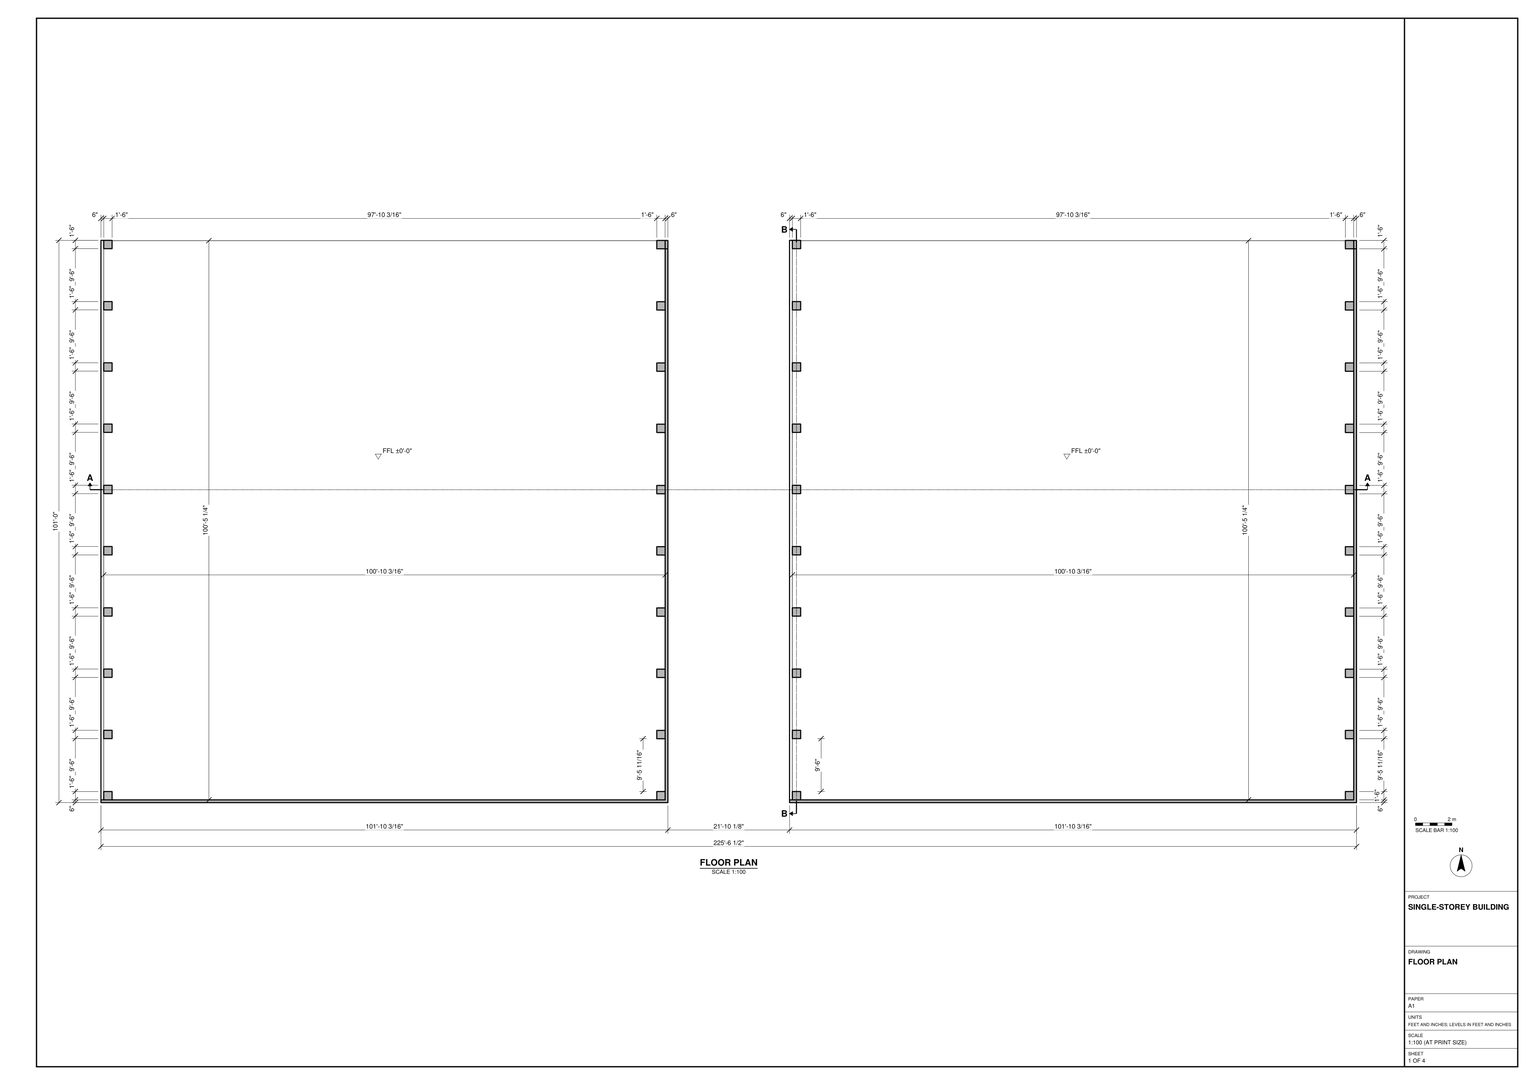
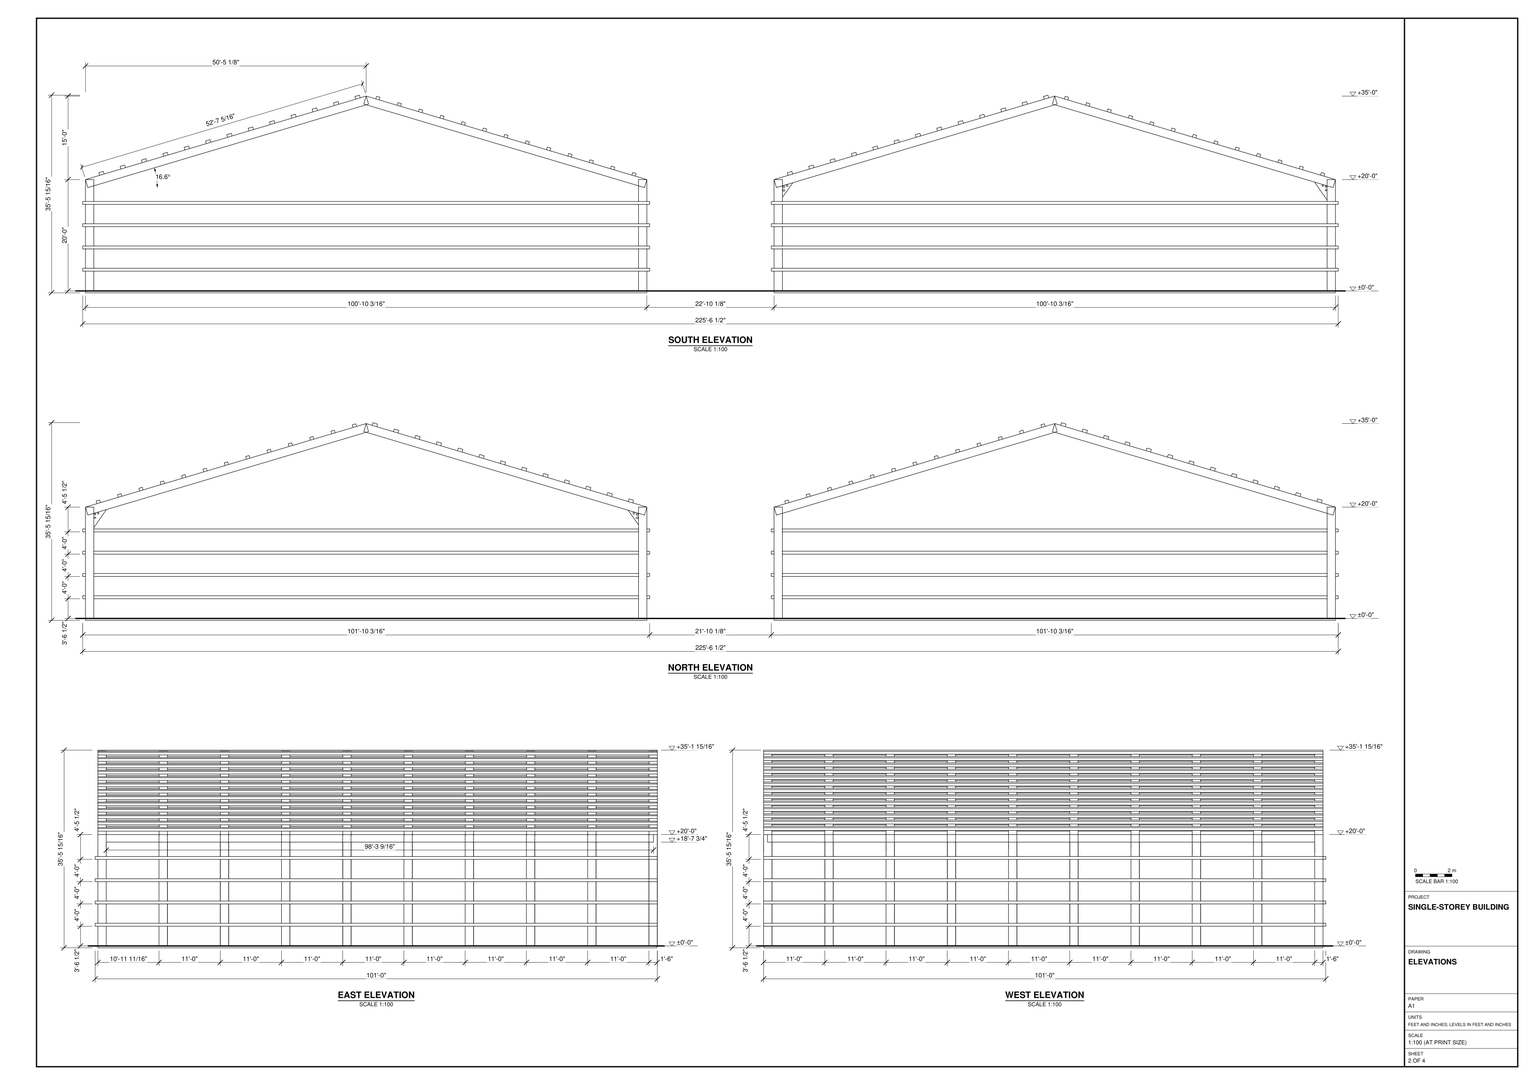
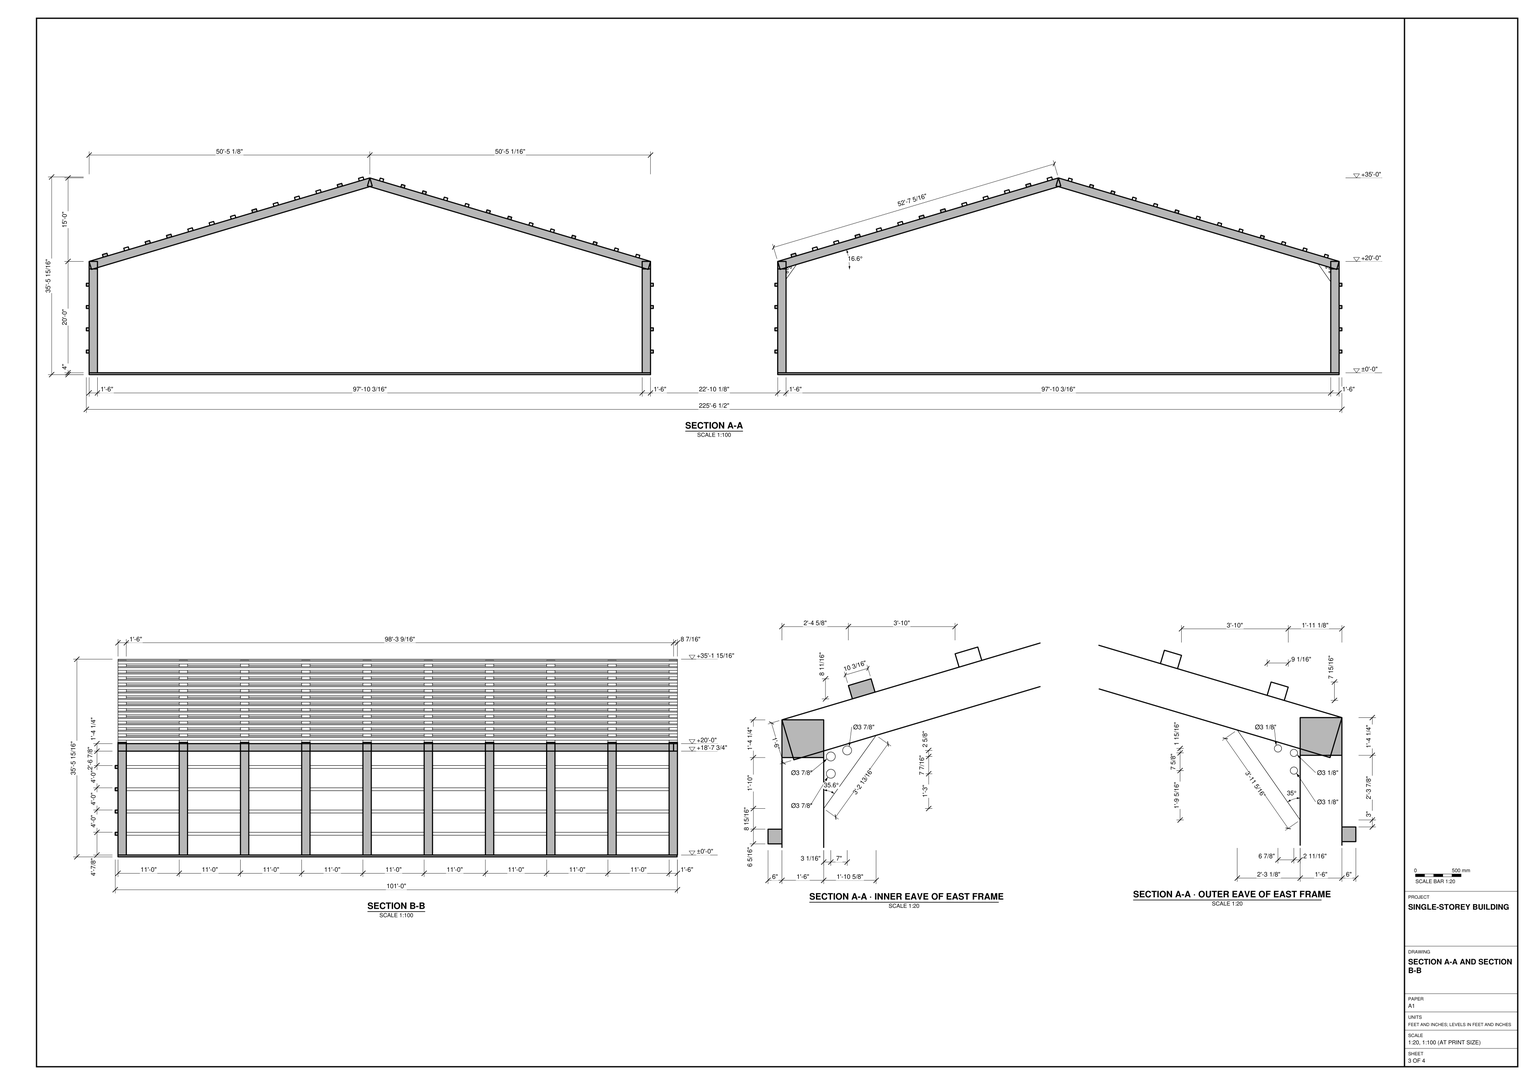
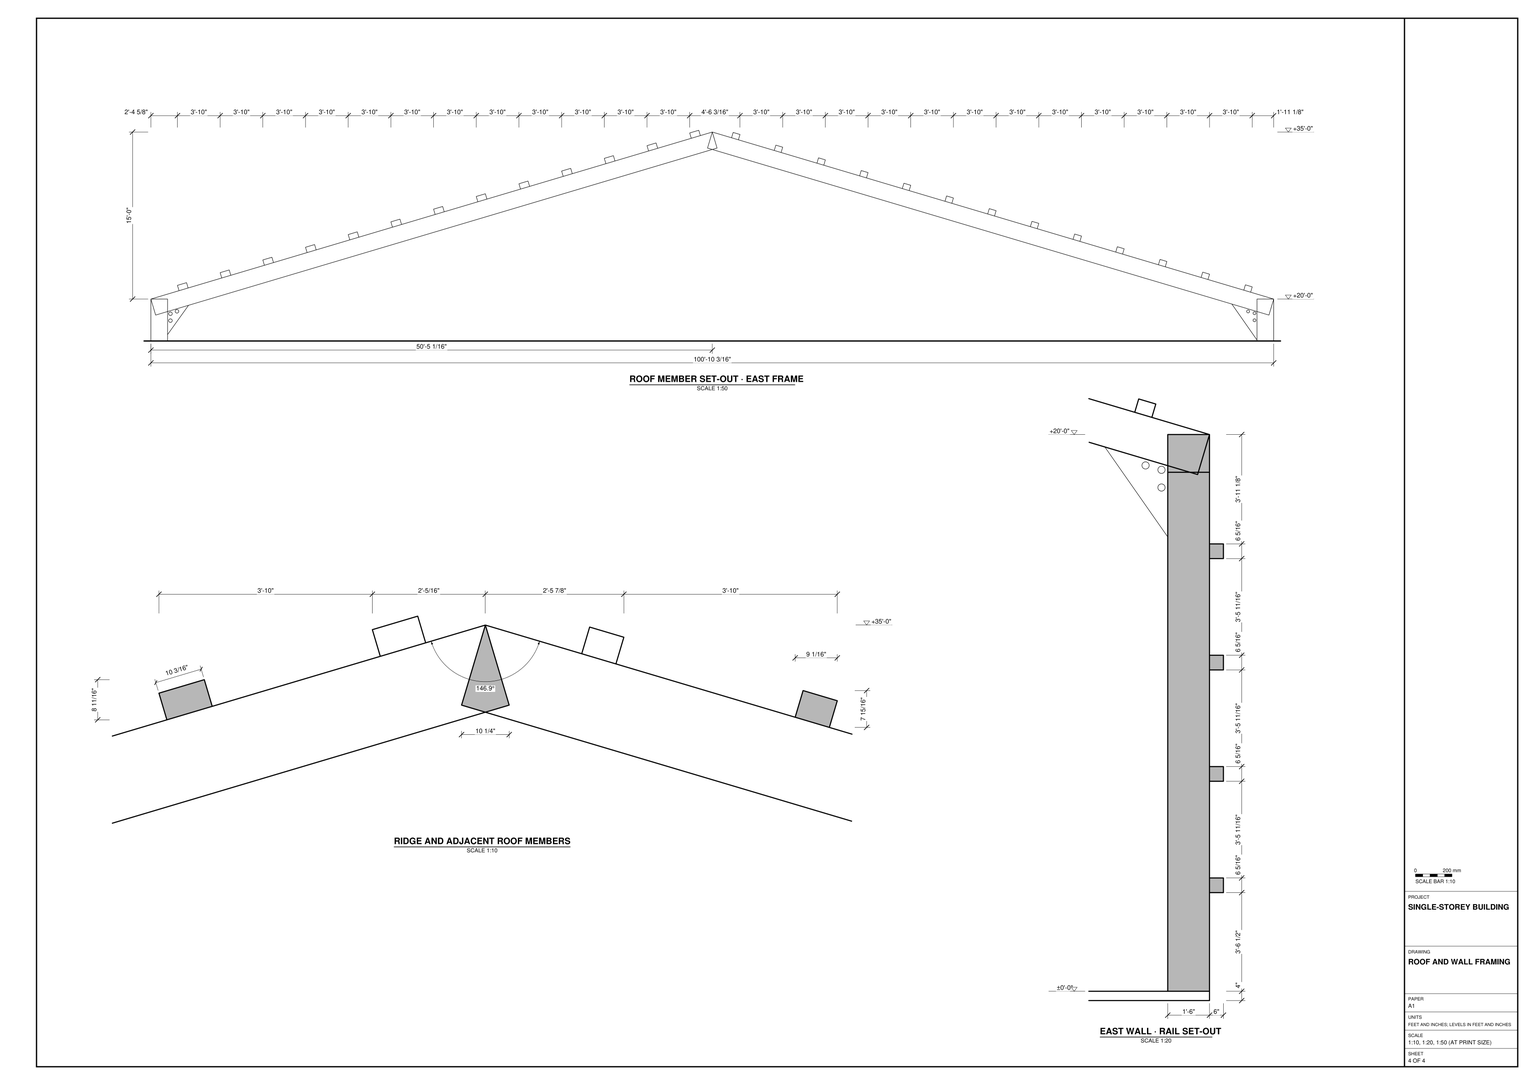
Build the two single-storey framed halls in SketchUp using task_files/diagram_01.pdf. Work in feet and inches. Set the finished floor of both halls at ±0'-0". The overall model must measure 225'-6 1/2" east to west, 101'-0" north to south and 35'-5 15/16" from its lowest to its highest point.

Lay out the two rectangular floor slabs side by side, with their north and south ends aligned. Leave the 21'-10 1/8" gap shown in plan between the halls. Keep each floor clear of interior partitions and columns. Along the east and west sides of each hall, place the paired columns at the bay spacing shown. Connect each pair with sloping rafters that meet at the ridge. Use the sections to size the framing and to distinguish the braced eave joints from the plain joints. Model the horizontal wall rails and the roof purlins as members with the cross-sections shown, leaving the spaces between them open.

Keep the slabs, wall framing and roof framing in separate groups or components, and use components for repeated members. Any decor or loose items shown may use suitable library components. Save one SketchUp model as output_files/two_single_storey_halls_with_exposed_gable_roof_framing.skp.

# SketchUp Ruby script. Lengths in inches.
U = 1.inch
M = Sketchup.active_model
def pt(a) = Geom::Point3d.new(a.map { |v| v * U })
def face(e, loops, mat)
  f = e.add_face(loops[0].map { |a| pt(a) })
  loops[1..].each { |l| e.add_face(l.map { |a| pt(a) }).erase! }
  f.material = f.back_material = mat if mat
  f
end
# faces: each face lists its corners as indices into pts; further lists are holes
def faces(e, pts, list, mat = nil) = list.each { |f| face(e, (f[0].is_a?(Array) ? f : [f]).map { |l| l.map { |i| pts[i] } }, mat) }
# xy, xz, yz: faces in a plane at the given z, y or x. An outline is a flat list of corners, or four numbers for a rectangle; further outlines are holes
def ring(l) = l.size == 4 ? [[l[0], l[1]], [l[2], l[1]], [l[2], l[3]], [l[0], l[3]]] : l.each_slice(2).to_a
def flat(e, list, mat, &to3) = list.each { |f| face(e, (f[0].is_a?(Array) ? f : [f]).map { |l| ring(l).map { |u, v| to3.(u, v) } }, mat) }
def xy(e, z, list, mat = nil) = flat(e, list, mat) { |x, y| [x, y, z] }
def xz(e, y, list, mat = nil) = flat(e, list, mat) { |x, z| [x, y, z] }
def yz(e, x, list, mat = nil) = flat(e, list, mat) { |y, z| [x, y, z] }
def lines(e, pts, list) = list.each { |a, b| e.add_line(pt(pts[a]), pt(pts[b])) }
# prism: a flat outline (further loops are holes) pulled along v
def prism(e, loops, v, mat = nil)
  f = face(e, loops, mat); d = Geom::Vector3d.new(v.map { |x| x * U })
  f.pushpull(f.normal.samedirection?(d) ? d.length : -d.length)
end
def box(e, o, s, mat = nil) = prism(e, [[o, [o[0] + s[0], o[1], o[2]], [o[0] + s[0], o[1] + s[1], o[2]], [o[0], o[1] + s[1], o[2]]]], [0, 0, s[2]], mat)
def at(x, y, z, deg = 0) = Geom::Transformation.translation(pt([x, y, z])) * Geom::Transformation.rotation(ORIGIN, Z_AXIS, deg.degrees)
def axes(o, x, y, z) = Geom::Transformation.new([*x, 0, *y, 0, *z, 0, *pt(o).to_a, 1])
def part(name) = M.definitions.add(name)
# library, detail: a bought-in or finely detailed component or shape, given as its bounding box
def library(name, o, s) = part(name).tap { |d| box(d.entities, o, s) }
def detail(e, o, s) = box(e.add_group.entities, o, s)
def put(e, d, t, mat = nil) = e.add_instance(d, t).tap { |i| i.material = mat if mat }
def group(e, t, mat = nil) = e.add_group.tap { |g| g.transformation = t; g.material = mat if mat }.entities
root = M.entities
M.materials.add("[Aluminum]").color = [179, 179, 179]
M.materials.add("[Terrazzo Tile Accent]").color = [224, 221, 217]
c1 = part("Group\#1")
box(c1.entities,[0,0,0],[1210.1875,1205.25,4])
c2 = part("Group\#2")
box(c2.entities,[0,0,0],[18,18,240])
c3 = part("Group\#3")
box(c3.entities,[0,0,0],[18,18,240])
c4 = part("Group\#4")
box(c4.entities,[0,0,0],[18,18,240])
c5 = part("Group\#5")
box(c5.entities,[0,0,0],[18,18,240])
c6 = part("Group\#6")
box(c6.entities,[0,0,0],[18,18,240])
c7 = part("Group\#7")
box(c7.entities,[0,0,0],[18,18,240])
c8 = part("Group\#8")
box(c8.entities,[0,0,0],[18,18,240])
c9 = part("Group\#9")
box(c9.entities,[0,0,0],[18,18,240])
c10 = part("Group\#10")
box(c10.entities,[0,0,0],[18,18,240])
c11 = part("Group\#11")
box(c11.entities,[0,0,0],[18,18,240])
c12 = part("Group\#12")
xz(c12.entities,0,[[5.13,0,605.09,178.47,599.96,180,605.09,197.25,0,17.25],[1205.06,0,1210.1875,17.25,605.09,197.25,610.23,180,605.09,178.47],[605.09,178.47,610.23,180,605.09,197.25,599.96,180]])
xz(c12.entities,18,[[5.13,0,0,17.25,605.09,197.25,599.96,180,605.09,178.47],[1205.06,0,605.09,178.47,610.23,180,605.09,197.25,1210.1875,17.25],[605.09,178.47,599.96,180,605.09,197.25,610.23,180]])
p = [[0,0,17.25],[0,18,17.25],[5.13,18,0],[5.13,0,0],[605.09,18,178.47],[610.23,18,180],
  [610.23,0,180],[605.09,0,178.47],[599.96,18,180],[1205.06,18,0],[1205.06,0,0],[599.96,0,180],
  [1210.1875,18,17.25],[1210.1875,0,17.25],[605.09,0,197.25],[605.09,18,197.25]]
faces(c12.entities,p,[[0,1,2,3],[3,2,4,5,6,7],[8,4,9,10,7,11],[12,13,10,9],[1,0,14,15],[12,15,14,13],[14,15,8,11],[15,14,6,5]])
c13 = part("Group\#13")
box(c13.entities,[0,0,0],[18,1179.59,16.27])
c14 = part("Group\#39")
prism(c14.entities,[[[1.71,1206,0],[1.71,0,0],[0,0,5.75],[0,1206,5.75]]],[9.78,0,2.91])
c15 = part("Group\#38")
prism(c15.entities,[[[1.71,1206,0],[1.71,0,0],[0,0,5.75],[0,1206,5.75]]],[9.78,0,2.91])
c16 = part("Group\#37")
prism(c16.entities,[[[1.71,1206,0],[1.71,0,0],[0,0,5.75],[0,1206,5.75]]],[9.78,0,2.91])
c17 = part("Group\#36")
prism(c17.entities,[[[1.71,1206,0],[1.71,0,0],[0,0,5.75],[0,1206,5.75]]],[9.78,0,2.91])
c18 = part("Group\#35")
prism(c18.entities,[[[1.71,1206,0],[1.71,0,0],[0,0,5.75],[0,1206,5.75]]],[9.78,0,2.91])
c19 = part("Group\#34")
prism(c19.entities,[[[1.71,1206,0],[1.71,0,0],[0,0,5.75],[0,1206,5.75]]],[9.78,0,2.91])
c20 = part("Group\#33")
prism(c20.entities,[[[1.71,1206,0],[1.71,0,0],[0,0,5.75],[0,1206,5.75]]],[9.78,0,2.91])
c21 = part("Group\#32")
prism(c21.entities,[[[1.71,1206,0],[1.71,0,0],[0,0,5.75],[0,1206,5.75]]],[9.78,0,2.91])
c22 = part("Group\#31")
prism(c22.entities,[[[1.71,1206,0],[1.71,0,0],[0,0,5.75],[0,1206,5.75]]],[9.78,0,2.91])
c23 = part("Group\#30")
prism(c23.entities,[[[1.71,1206,0],[1.71,0,0],[0,0,5.75],[0,1206,5.75]]],[9.78,0,2.91])
c24 = part("Group\#29")
prism(c24.entities,[[[1.71,1206,0],[1.71,0,0],[0,0,5.75],[0,1206,5.75]]],[9.78,0,2.91])
c25 = part("Group\#28")
prism(c25.entities,[[[1.71,1206,0],[1.71,0,0],[0,0,5.75],[0,1206,5.75]]],[9.78,0,2.91])
c26 = part("Group\#14")
prism(c26.entities,[[[1.71,1206,0],[1.71,0,0],[0,0,5.75],[0,1206,5.75]]],[9.78,0,2.91])
c27 = part("Group\#15")
prism(c27.entities,[[[0,1206,2.19],[7.37,1206,0],[7.37,0,0],[0,0,2.19]]],[1.71,0,5.75])
c28 = part("Group\#16")
prism(c28.entities,[[[0,1206,2.19],[7.37,1206,0],[7.37,0,0],[0,0,2.19]]],[1.71,0,5.75])
c29 = part("Group\#17")
prism(c29.entities,[[[0,1206,2.19],[7.37,1206,0],[7.37,0,0],[0,0,2.19]]],[1.71,0,5.75])
c30 = part("Group\#18")
prism(c30.entities,[[[0,1206,2.19],[7.37,1206,0],[7.37,0,0],[0,0,2.19]]],[1.71,0,5.75])
c31 = part("Group\#19")
prism(c31.entities,[[[0,1206,2.19],[7.37,1206,0],[7.37,0,0],[0,0,2.19]]],[1.71,0,5.75])
c32 = part("Group\#20")
prism(c32.entities,[[[0,1206,2.19],[7.37,1206,0],[7.37,0,0],[0,0,2.19]]],[1.71,0,5.75])
c33 = part("Group\#21")
prism(c33.entities,[[[0,1206,2.19],[7.37,1206,0],[7.37,0,0],[0,0,2.19]]],[1.71,0,5.75])
c34 = part("Group\#22")
prism(c34.entities,[[[0,1206,2.19],[7.37,1206,0],[7.37,0,0],[0,0,2.19]]],[1.71,0,5.75])
c35 = part("Group\#23")
prism(c35.entities,[[[0,1206,2.19],[7.37,1206,0],[7.37,0,0],[0,0,2.19]]],[1.71,0,5.75])
c36 = part("Group\#24")
prism(c36.entities,[[[0,1206,2.19],[7.37,1206,0],[7.37,0,0],[0,0,2.19]]],[1.71,0,5.75])
c37 = part("Group\#25")
prism(c37.entities,[[[0,1206,2.19],[7.37,1206,0],[7.37,0,0],[0,0,2.19]]],[1.71,0,5.75])
c38 = part("Group\#26")
prism(c38.entities,[[[0,1206,2.19],[7.37,1206,0],[7.37,0,0],[0,0,2.19]]],[1.71,0,5.75])
c39 = part("Group\#27")
prism(c39.entities,[[[0,1206,2.19],[7.37,1206,0],[7.37,0,0],[0,0,2.19]]],[1.71,0,5.75])
c40 = part("Group\#40")
yz(c40.entities,0,[[0,0,18,6.33]])
c41 = part("Group\#49")
g1 = group(c41.entities,at(0,0,0))
xy(g1,0,[[0,0,6,18]])
xy(g1,6.33,[[0,0,6,18]])
xz(g1,0,[[0,0,6,6.33]])
xz(g1,18,[[0,0,6,6.33]])
yz(g1,0,[[0,0,18,6.33]])
put(c41.entities,c40,at(6,0,0))
c42 = part("Group\#51")
g2 = group(c42.entities,at(0,0,0))
xy(g2,0,[[0,0,6,18]])
xy(g2,6.33,[[0,0,6,18]])
xz(g2,0,[[0,0,6,6.33]])
xz(g2,18,[[0,0,6,6.33]])
yz(g2,0,[[0,0,18,6.33]])
put(c42.entities,c40,at(6,0,0))
c43 = part("Group\#53")
g3 = group(c43.entities,at(0,0,0))
xy(g3,0,[[0,0,6,18]])
xy(g3,6.33,[[0,0,6,18]])
xz(g3,0,[[0,0,6,6.33]])
xz(g3,18,[[0,0,6,6.33]])
yz(g3,0,[[0,0,18,6.33]])
put(c43.entities,c40,at(6,0,0))
c44 = part("Group\#42")
g4 = group(c44.entities,at(0,0,0))
xy(g4,0,[[0,-1188,6,18]])
xy(g4,6.33,[[0,-1188,6,18]])
xz(g4,-1188,[[0,0,6,6.33]])
xz(g4,18,[[0,0,6,6.33]])
yz(g4,0,[[-1188,0,18,6.33]])
put(c44.entities,c40,at(6,0,0))
c45 = part("Group\#43")
g5 = group(c45.entities,at(0,0,0))
xy(g5,0,[[0,-1188,6,18]])
xy(g5,6.33,[[0,-1188,6,18]])
xz(g5,-1188,[[0,0,6,6.33]])
xz(g5,18,[[0,0,6,6.33]])
yz(g5,0,[[-1188,0,18,6.33]])
put(c45.entities,c40,at(6,0,0))
c46 = part("Group\#45")
g6 = group(c46.entities,at(0,0,0))
xy(g6,0,[[0,-1188,6,18]])
xy(g6,6.33,[[0,-1188,6,18]])
xz(g6,-1188,[[0,0,6,6.33]])
xz(g6,18,[[0,0,6,6.33]])
yz(g6,0,[[-1188,0,18,6.33]])
put(c46.entities,c40,at(6,0,0))
c47 = part("Group\#47")
g7 = group(c47.entities,at(0,0,0))
xy(g7,0,[[0,-1188,6,18]])
xy(g7,6.33,[[0,-1188,6,18]])
xz(g7,-1188,[[0,0,6,6.33]])
xz(g7,18,[[0,0,6,6.33]])
yz(g7,0,[[-1188,0,18,6.33]])
put(c47.entities,c40,at(6,0,0))
c48 = part("Group\#55")
p = [[27.12,0,30.73],[27.12,0,0],[0,0.28,38.8],[24.42,0.03,27.37],[24.82,0.02,27.43],[25.2,0.02,27.58],
  [25.52,0.02,27.83],[25.77,0.01,28.15],[25.93,0.01,28.53],[25.98,0.01,28.93],[25.93,0.01,29.34],[25.77,0.01,29.72],
  [25.52,0.02,30.04],[25.2,0.02,30.29],[24.82,0.02,30.44],[24.42,0.03,30.5],[24.01,0.03,30.44],[23.64,0.04,30.29],
  [23.3125,0.04,30.04],[23.06,0.04,29.72],[22.91,0.04,29.34],[22.86,0.04,28.93],[22.91,0.04,28.53],[23.06,0.04,28.15],
  [23.3125,0.04,27.83],[23.64,0.04,27.58],[24.01,0.03,27.43],[16.04,0.12,31.25],[15.99,0.12,30.84],[16.04,0.12,30.4375],
  [16.2,0.11,30.0625],[16.45,0.11,29.74],[16.77,0.11,29.49],[17.15,0.1,29.33],[17.55,0.1,29.28],[17.96,0.1,29.33],
  [18.33,0.09,29.49],[18.66,0.09,29.74],[18.91,0.09,30.0625],[19.0625,0.08,30.4375],[19.12,0.08,30.84],[19.0625,0.08,31.25],
  [18.91,0.09,31.625],[18.66,0.09,31.95],[18.33,0.09,32.2],[17.96,0.1,32.35],[17.55,0.1,32.4],[17.15,0.1,32.35],
  [16.77,0.11,32.2],[16.45,0.11,31.95],[16.2,0.11,31.625],[22.91,0.04,21.71],[22.86,0.04,21.31],[22.91,0.04,20.91],
  [23.06,0.04,20.53],[23.3125,0.04,20.2],[23.64,0.04,19.96],[24.01,0.03,19.8],[24.42,0.03,19.75],[24.82,0.02,19.8],
  [25.2,0.02,19.96],[25.52,0.02,20.2],[25.77,0.01,20.53],[25.93,0.01,20.91],[25.98,0.01,21.31],[25.93,0.01,21.71],
  [25.77,0.01,22.09],[25.52,0.02,22.41],[25.2,0.02,22.66],[24.82,0.02,22.82],[24.42,0.03,22.87],[24.01,0.03,22.82],
  [23.64,0.04,22.66],[23.3125,0.04,22.41],[23.06,0.04,22.09]]
faces(c48.entities,p,[[[0,1,2],[3,4,5,6,7,8,9,10,11,12,13,14,15,16,17,18,19,20,21,22,23,24,25,26],[27,28,29,30,31,32,33,34,35,36,37,38,39,40,41,42,43,44,45,46,47,48,49,50],[51,52,53,54,55,56,57,58,59,60,61,62,63,64,65,66,67,68,69,70,71,72,73,74]],[59,58,57,56,55,54,53,52,51,74,73,72,71,70,69,68,67,66,65,64,63,62,61,60],[4,3,26,25,24,23,22,21,20,19,18,17,16,15,14,13,12,11,10,9,8,7,6,5],[35,34,33,32,31,30,29,28,27,50,49,48,47,46,45,44,43,42,41,40,39,38,37,36]])
c49 = part("Group\#56")
xz(c49.entities,0,[[[0,0,0,24.82,22.6,31.54],[3.15,20.51,3.65,20.59,4.11,20.8,4.5,21.12,4.79,21.53,4.97,22,5.02,22.51,4.93,23.01,4.73,23.47,4.4,23.86,3.99,24.15,3.52,24.33,3.02,24.38,2.52,24.3,2.06,24.09,1.67,23.77,1.37,23.35,1.19,22.88,1.14,22.38,1.23,21.88,1.4375,21.42,1.76,21.03,2.17,20.73,2.64,20.56],[3.15,13.07,3.65,13.15,4.11,13.36,4.5,13.68,4.79,14.09,4.97,14.57,5.02,15.07,4.93,15.57,4.73,16.03,4.4,16.42,3.99,16.71,3.52,16.89,3.02,16.94,2.52,16.86,2.06,16.65,1.67,16.33,1.37,15.92,1.19,15.44,1.14,14.94,1.23,14.44,1.4375,13.98,1.76,13.59,2.17,13.3,2.64,13.12],[10.18,23.12,10.67,23.21,11.13,23.42,11.53,23.74,11.82,24.15,12,24.62,12.05,25.125,11.96,25.625,11.75,26.08,11.43,26.47,11.02,26.77,10.55,26.95,10.04,27,9.55,26.91,9.08,26.7,8.69,26.38,8.4,25.97,8.22,25.5,8.17,24.99,8.26,24.49,8.47,24.03,8.79,23.64,9.2,23.35,9.67,23.17]],[3.15,13.07,2.64,13.12,2.17,13.3,1.76,13.59,1.4375,13.98,1.23,14.44,1.14,14.94,1.19,15.44,1.37,15.92,1.67,16.33,2.06,16.65,2.52,16.86,3.02,16.94,3.52,16.89,3.99,16.71,4.4,16.42,4.73,16.03,4.93,15.57,5.02,15.07,4.97,14.57,4.79,14.09,4.5,13.68,4.11,13.36,3.65,13.15],[3.15,20.51,2.64,20.56,2.17,20.73,1.76,21.03,1.4375,21.42,1.23,21.88,1.14,22.38,1.19,22.88,1.37,23.35,1.67,23.77,2.06,24.09,2.52,24.3,3.02,24.38,3.52,24.33,3.99,24.15,4.4,23.86,4.73,23.47,4.93,23.01,5.02,22.51,4.97,22,4.79,21.53,4.5,21.12,4.11,20.8,3.65,20.59],[10.18,23.12,9.67,23.17,9.2,23.35,8.79,23.64,8.47,24.03,8.26,24.49,8.17,24.99,8.22,25.5,8.4,25.97,8.69,26.38,9.08,26.7,9.55,26.91,10.04,27,10.55,26.95,11.02,26.77,11.43,26.47,11.75,26.08,11.96,25.625,12.05,25.125,12,24.62,11.82,24.15,11.53,23.74,11.13,23.42,10.67,23.21]])
xy(root,46.52,[[0,0,0,6,1216.1875,6,1216.1875,1193.72,1222.1875,1193.72,1222.1875,0],[1484.3125,0,1484.3125,6,2700.5,6,2700.5,1193.72,2706.5,1193.72,2706.5,0]])
xy(root,52.85,[[1484.3125,0,2706.5,0,2706.5,1193.72,2700.5,1193.72,2700.5,6,1484.3125,6]])
xy(root,52.85,[[0,0,1222.1875,0,1222.1875,1193.72,1216.1875,1193.72,1216.1875,6,0,6]],"[Aluminum]")
xy(root,94.52,[[0,0,0,6,1216.1875,6,1216.1875,1193.72,1222.1875,1193.72,1222.1875,0],[1484.3125,0,1484.3125,6,2700.5,6,2700.5,1193.72,2706.5,1193.72,2706.5,0]])
xy(root,100.85,[[1484.3125,0,2706.5,0,2706.5,1193.72,2700.5,1193.72,2700.5,6,1484.3125,6]])
xy(root,100.85,[[0,0,1222.1875,0,1222.1875,1193.72,1216.1875,1193.72,1216.1875,6,0,6]],"[Aluminum]")
xy(root,142.52,[[0,0,0,6,1216.1875,6,1216.1875,1193.72,1222.1875,1193.72,1222.1875,0],[1484.3125,0,1484.3125,6,2700.5,6,2700.5,1193.72,2706.5,1193.72,2706.5,0]])
xy(root,148.85,[[1484.3125,0,2706.5,0,2706.5,1193.72,2700.5,1193.72,2700.5,6,1484.3125,6]])
xy(root,148.85,[[0,0,1222.1875,0,1222.1875,1193.72,1216.1875,1193.72,1216.1875,6,0,6]],"[Aluminum]")
xy(root,190.52,[[0,0,0,6,1216.1875,6,1216.1875,1193.72,1222.1875,1193.72,1222.1875,0],[1484.3125,0,1484.3125,6,2700.5,6,2700.5,1193.72,2706.5,1193.72,2706.5,0]])
xy(root,196.85,[[1484.3125,0,2706.5,0,2706.5,1193.72,2700.5,1193.72,2700.5,6,1484.3125,6]])
xy(root,196.85,[[0,0,1222.1875,0,1222.1875,1193.72,1216.1875,1193.72,1216.1875,6,0,6]],"[Aluminum]")
xz(root,0,[[0,46.52,1222.1875,52.85],[1484.3125,46.52,2706.5,52.85],[0,94.52,1222.1875,100.85],[1484.3125,94.52,2706.5,100.85],[0,142.52,1222.1875,148.85],
  [1484.3125,142.52,2706.5,148.85],[0,190.52,1222.1875,196.85],[1484.3125,190.52,2706.5,196.85]],"[Aluminum]")
xz(root,6,[[0,46.52,1216.1875,52.85],[1484.3125,46.52,2700.5,52.85],[0,94.52,1216.1875,100.85],[1484.3125,94.52,2700.5,100.85],[0,142.52,1216.1875,148.85],
  [1484.3125,142.52,2700.5,148.85],[0,190.52,1216.1875,196.85],[1484.3125,190.52,2700.5,196.85]])
xz(root,1193.72,[[1216.1875,46.52,1222.1875,52.85],[2700.5,46.52,2706.5,52.85],[1216.1875,94.52,1222.1875,100.85],[2700.5,94.52,2706.5,100.85],[1216.1875,142.52,1222.1875,148.85],
  [2700.5,142.52,2706.5,148.85],[1216.1875,190.52,1222.1875,196.85],[2700.5,190.52,2706.5,196.85]])
yz(root,0,[[0,46.52,6,52.85],[0,94.52,6,100.85],[0,142.52,6,148.85],[0,190.52,6,196.85]])
yz(root,1216.1875,[[6,46.52,1193.72,52.85],[6,94.52,1193.72,100.85],[6,142.52,1193.72,148.85],[6,190.52,1193.72,196.85]])
yz(root,1222.1875,[[0,46.52,1193.72,52.85],[0,94.52,1193.72,100.85],[0,142.52,1193.72,148.85],[0,190.52,1193.72,196.85]],"[Aluminum]")
yz(root,1484.3125,[[0,46.52,6,52.85],[0,94.52,6,100.85],[0,142.52,6,148.85],[0,190.52,6,196.85]])
yz(root,2700.5,[[6,46.52,1193.72,52.85],[6,94.52,1193.72,100.85],[6,142.52,1193.72,148.85],[6,190.52,1193.72,196.85]])
yz(root,2706.5,[[0,46.52,1193.72,52.85],[0,94.52,1193.72,100.85],[0,142.52,1193.72,148.85],[0,190.52,1193.72,196.85]],"[Aluminum]")
put(root,c1,at(1490.3125,6,0),"[Terrazzo Tile Accent]")
put(root,c2,at(1490.3125,6,4),"[Aluminum]")
put(root,c3,at(1490.3125,138,4),"[Aluminum]")
put(root,c4,at(1490.3125,270,4),"[Aluminum]")
put(root,c5,at(1490.3125,402,4),"[Aluminum]")
put(root,c6,at(1490.3125,534,4),"[Aluminum]")
put(root,c7,at(1490.3125,666,4),"[Aluminum]")
put(root,c8,at(1490.3125,798,4),"[Aluminum]")
put(root,c9,at(1490.3125,930,4),"[Aluminum]")
put(root,c10,at(1490.3125,1062,4),"[Aluminum]")
put(root,c11,at(1490.3125,1194,4),"[Aluminum]")
put(root,c2,at(2682.5,6,4),"[Aluminum]")
put(root,c2,at(2682.5,137.72,4),"[Aluminum]")
put(root,c2,at(2682.5,269.72,4),"[Aluminum]")
put(root,c2,at(2682.5,401.72,4),"[Aluminum]")
put(root,c2,at(2682.5,533.72,4),"[Aluminum]")
put(root,c2,at(2682.5,665.72,4),"[Aluminum]")
put(root,c2,at(2682.5,797.72,4),"[Aluminum]")
put(root,c2,at(2682.5,929.72,4),"[Aluminum]")
put(root,c2,at(2682.5,1061.72,4),"[Aluminum]")
put(root,c2,at(2682.5,1193.72,4),"[Aluminum]")
put(root,c12,at(1490.3125,6,226.75),"[Aluminum]")
put(root,c12,at(1490.3125,138,226.75),"[Aluminum]")
put(root,c12,at(1490.3125,270,226.75),"[Aluminum]")
put(root,c12,at(1490.3125,402,226.75),"[Aluminum]")
put(root,c12,at(1490.3125,534,226.75),"[Aluminum]")
put(root,c12,at(1490.3125,666,226.75),"[Aluminum]")
put(root,c12,at(1490.3125,798,226.75),"[Aluminum]")
put(root,c12,at(1490.3125,930,226.75),"[Aluminum]")
put(root,c12,at(1490.3125,1062,226.75),"[Aluminum]")
put(root,c12,at(1490.3125,1194,226.75),"[Aluminum]")
put(root,c13,at(1490.3125,24,227.73),"[Aluminum]")
put(root,c13,at(2682.5,24,227.73),"[Aluminum]")
put(root,c14,at(1518.96,6,253.03),"[Aluminum]")
put(root,c15,at(1564.96,6,266.72),"[Aluminum]")
put(root,c16,at(1610.97,6,280.4),"[Aluminum]")
put(root,c17,at(1656.98,6,294.09),"[Aluminum]")
put(root,c18,at(1702.99,6,307.77),"[Aluminum]")
put(root,c19,at(1748.99,6,321.46),"[Aluminum]")
put(root,c20,at(1795,6,335.15),"[Aluminum]")
put(root,c21,at(1841.01,6,348.83),"[Aluminum]")
put(root,c22,at(1887.02,6,362.52),"[Aluminum]")
put(root,c23,at(1933.02,6,376.2),"[Aluminum]")
put(root,c24,at(1979.03,6,389.89),"[Aluminum]")
put(root,c25,at(2025.04,6,403.58),"[Aluminum]")
put(root,c26,at(2071.05,6,417.26),"[Aluminum]")
put(root,c27,at(2668.27,6,251.4),"[Aluminum]")
put(root,c28,at(2622.26,6,265.08),"[Aluminum]")
put(root,c29,at(2576.25,6,278.77),"[Aluminum]")
put(root,c30,at(2530.24,6,292.45),"[Aluminum]")
put(root,c31,at(2484.24,6,306.14),"[Aluminum]")
put(root,c32,at(2438.23,6,319.83),"[Aluminum]")
put(root,c33,at(2392.22,6,333.51),"[Aluminum]")
put(root,c34,at(2346.21,6,347.2),"[Aluminum]")
put(root,c35,at(2300.21,6,360.88),"[Aluminum]")
put(root,c36,at(2254.2,6,374.57),"[Aluminum]")
put(root,c37,at(2208.19,6,388.26),"[Aluminum]")
put(root,c38,at(2162.18,6,401.94),"[Aluminum]")
put(root,c39,at(2116.18,6,415.63),"[Aluminum]")
put(root,c41,at(2700.5,1193.72,190.52),"[Aluminum]")
put(root,c42,at(2700.5,1193.72,142.52),"[Aluminum]")
put(root,c43,at(2700.5,1193.72,94.52),"[Aluminum]")
put(root,c43,at(2700.5,1193.72,46.52),"[Aluminum]")
put(root,c44,at(1484.3125,1194,190.52),"[Aluminum]")
put(root,c45,at(1484.3125,1194,142.52),"[Aluminum]")
put(root,c46,at(1484.3125,1194,94.52),"[Aluminum]")
put(root,c47,at(1484.3125,1194,46.52),"[Aluminum]")
put(root,c6,at(6,534,4),"[Aluminum]")
put(root,c4,at(6,270,4),"[Aluminum]")
put(root,c2,at(6,6,4),"[Aluminum]")
put(root,c22,at(402.7,6,362.52),"[Aluminum]")
put(root,c7,at(6,666,4),"[Aluminum]")
put(root,c19,at(264.68,6,321.46),"[Aluminum]")
put(root,c13,at(6,24,227.73),"[Aluminum]")
put(root,c9,at(6,930,4),"[Aluminum]")
put(root,c3,at(6,138,4),"[Aluminum]")
put(root,c10,at(6,1062,4),"[Aluminum]")
put(root,c18,at(218.67,6,307.77),"[Aluminum]")
put(root,c11,at(6,1194,4),"[Aluminum]")
put(root,c8,at(6,798,4),"[Aluminum]")
put(root,c1,at(6,6,0),"[Terrazzo Tile Accent]")
put(root,c20,at(310.6875,6,335.15),"[Aluminum]")
put(root,c25,at(540.73,6,403.58),"[Aluminum]")
put(root,c12,at(6,666,226.75),"[Aluminum]")
put(root,c14,at(34.64,6,253.03),"[Aluminum]")
put(root,c23,at(448.71,6,376.2),"[Aluminum]")
put(root,c26,at(586.73,6,417.26),"[Aluminum]")
put(root,c15,at(80.65,6,266.72),"[Aluminum]")
put(root,c5,at(6,402,4),"[Aluminum]")
put(root,c24,at(494.72,6,389.89),"[Aluminum]")
put(root,c45,at(0,1194,142.52),"[Aluminum]")
put(root,c37,at(723.88,6,388.26),"[Aluminum]")
put(root,c2,at(1198.1875,929.72,4),"[Aluminum]")
put(root,c30,at(1045.93,6,292.45),"[Aluminum]")
put(root,c2,at(1198.1875,401.72,4),"[Aluminum]")
put(root,c32,at(953.92,6,319.83),"[Aluminum]")
put(root,c33,at(907.91,6,333.51),"[Aluminum]")
put(root,c28,at(1137.95,6,265.08),"[Aluminum]")
put(root,c12,at(6,402,226.75),"[Aluminum]")
put(root,c27,at(1183.95,6,251.4),"[Aluminum]")
put(root,c2,at(1198.1875,797.72,4),"[Aluminum]")
put(root,c2,at(1198.1875,1193.72,4),"[Aluminum]")
put(root,c34,at(861.9,6,347.2),"[Aluminum]")
put(root,c36,at(769.89,6,374.57),"[Aluminum]")
put(root,c2,at(1198.1875,533.72,4),"[Aluminum]")
put(root,c35,at(815.89,6,360.88),"[Aluminum]")
put(root,c2,at(1198.1875,665.72,4),"[Aluminum]")
put(root,c47,at(0,1194,46.52),"[Aluminum]")
put(root,c12,at(6,534,226.75),"[Aluminum]")
put(root,c44,at(0,1194,190.52),"[Aluminum]")
put(root,c2,at(1198.1875,1061.72,4),"[Aluminum]")
put(root,c38,at(677.87,6,401.94),"[Aluminum]")
put(root,c46,at(0,1194,94.52),"[Aluminum]")
put(root,c12,at(6,930,226.75),"[Aluminum]")
put(root,c12,at(6,1194,226.75),"[Aluminum]")
put(root,c16,at(126.66,6,280.4),"[Aluminum]")
put(root,c12,at(6,270,226.75),"[Aluminum]")
put(root,c12,at(6,138,226.75),"[Aluminum]")
put(root,c12,at(6,1062,226.75),"[Aluminum]")
put(root,c2,at(1198.1875,269.72,4),"[Aluminum]")
put(root,c2,at(1198.1875,6,4),"[Aluminum]")
put(root,c13,at(1198.1875,24,227.73),"[Aluminum]")
put(root,c39,at(631.86,6,415.63),"[Aluminum]")
put(root,c21,at(356.7,6,348.83),"[Aluminum]")
put(root,c31,at(999.92,6,306.14),"[Aluminum]")
put(root,c12,at(6,798,226.75),"[Aluminum]")
put(root,c29,at(1091.9375,6,278.77),"[Aluminum]")
put(root,c2,at(1198.1875,137.72,4),"[Aluminum]")
put(root,c42,at(1216.1875,1193.72,142.52),"[Aluminum]")
put(root,c43,at(1216.1875,1193.72,94.52),"[Aluminum]")
put(root,c17,at(172.67,6,294.09),"[Aluminum]")
put(root,c41,at(1216.1875,1193.72,190.52),"[Aluminum]")
put(root,c43,at(1216.1875,1193.72,46.52),"[Aluminum]")
put(root,c12,at(6,6,226.75),"[Aluminum]")
put(root,c48,at(2655.38,1211.72,199.84),"[Aluminum]")
put(root,c48,at(2655.38,1079.72,199.84),"[Aluminum]")
put(root,c48,at(2655.38,947.72,199.84),"[Aluminum]")
put(root,c48,at(2655.38,815.72,199.84),"[Aluminum]")
put(root,c48,at(2655.38,683.72,199.84),"[Aluminum]")
put(root,c48,at(2655.38,551.72,199.84),"[Aluminum]")
put(root,c48,at(2655.38,419.72,199.84),"[Aluminum]")
put(root,c48,at(2655.38,287.72,199.84),"[Aluminum]")
put(root,c48,at(2655.38,155.72,199.84),"[Aluminum]")
put(root,c48,at(2655.38,23.72,199.84),"[Aluminum]")
put(root,c49,at(1508.3125,1212,205.76),"[Aluminum]")
put(root,c49,at(1508.3125,1080,205.76),"[Aluminum]")
put(root,c49,at(1508.3125,948,205.76),"[Aluminum]")
put(root,c49,at(1508.3125,816,205.76),"[Aluminum]")
put(root,c49,at(1508.3125,684,205.76),"[Aluminum]")
put(root,c49,at(1508.3125,552,205.76),"[Aluminum]")
put(root,c49,at(1508.3125,420,205.76),"[Aluminum]")
put(root,c49,at(1508.3125,288,205.76),"[Aluminum]")
put(root,c49,at(1508.3125,156,205.76),"[Aluminum]")
put(root,c49,at(1508.3125,24,205.76),"[Aluminum]")
